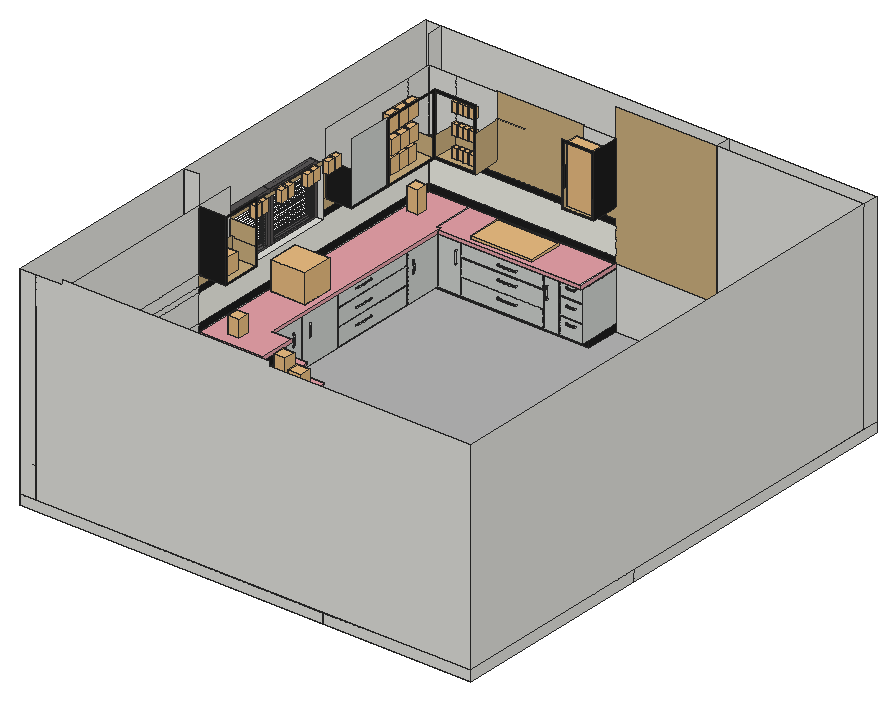
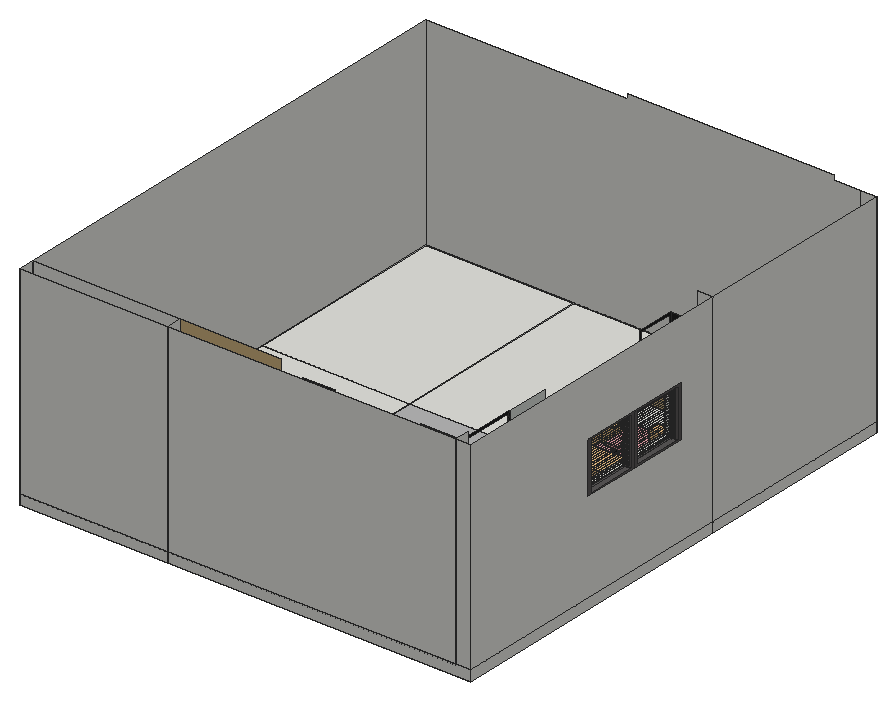
# SketchUp Ruby script. Lengths in inches.
U = 1.inch
M = Sketchup.active_model
def pt(a) = Geom::Point3d.new(a.map { |v| v * U })
def face(e, loops, mat)
  f = e.add_face(loops[0].map { |a| pt(a) })
  loops[1..].each { |l| e.add_face(l.map { |a| pt(a) }).erase! }
  f.material = f.back_material = mat if mat
  f
end
# faces: each face lists its corners as indices into pts; further lists are holes
def faces(e, pts, list, mat = nil) = list.each { |f| face(e, (f[0].is_a?(Array) ? f : [f]).map { |l| l.map { |i| pts[i] } }, mat) }
# xy, xz, yz: faces in a plane at the given z, y or x. An outline is a flat list of corners, or four numbers for a rectangle; further outlines are holes
def ring(l) = l.size == 4 ? [[l[0], l[1]], [l[2], l[1]], [l[2], l[3]], [l[0], l[3]]] : l.each_slice(2).to_a
def flat(e, list, mat, &to3) = list.each { |f| face(e, (f[0].is_a?(Array) ? f : [f]).map { |l| ring(l).map { |u, v| to3.(u, v) } }, mat) }
def xy(e, z, list, mat = nil) = flat(e, list, mat) { |x, y| [x, y, z] }
def xz(e, y, list, mat = nil) = flat(e, list, mat) { |x, z| [x, y, z] }
def yz(e, x, list, mat = nil) = flat(e, list, mat) { |y, z| [x, y, z] }
def lines(e, pts, list) = list.each { |a, b| e.add_line(pt(pts[a]), pt(pts[b])) }
# prism: a flat outline (further loops are holes) pulled along v
def prism(e, loops, v, mat = nil)
  f = face(e, loops, mat); d = Geom::Vector3d.new(v.map { |x| x * U })
  f.pushpull(f.normal.samedirection?(d) ? d.length : -d.length)
end
def box(e, o, s, mat = nil) = prism(e, [[o, [o[0] + s[0], o[1], o[2]], [o[0] + s[0], o[1] + s[1], o[2]], [o[0], o[1] + s[1], o[2]]]], [0, 0, s[2]], mat)
def at(x, y, z, deg = 0) = Geom::Transformation.translation(pt([x, y, z])) * Geom::Transformation.rotation(ORIGIN, Z_AXIS, deg.degrees)
def axes(o, x, y, z) = Geom::Transformation.new([*x, 0, *y, 0, *z, 0, *pt(o).to_a, 1])
def part(name) = M.definitions.add(name)
# library, detail: a bought-in or finely detailed component or shape, given as its bounding box
def library(name, o, s) = part(name).tap { |d| box(d.entities, o, s) }
def detail(e, o, s) = box(e.add_group.entities, o, s)
def put(e, d, t, mat = nil) = e.add_instance(d, t).tap { |i| i.material = mat if mat }
def group(e, t, mat = nil) = e.add_group.tap { |g| g.transformation = t; g.material = mat if mat }.entities
root = M.entities
M.materials.add("Emissive").color = [223, 214, 154]
M.materials.add("GLASS BLADE REFRACTION").color = [24, 24, 24]
M.materials["GLASS BLADE REFRACTION"].alpha = 0.5
M.materials.add("Generic").color = [208, 212, 208]
M.materials.add("JalousieFrame").color = [89, 86, 86]
M.materials.add("Tiles Simple 02 100cm").color = [183, 183, 183]
M.materials.add("W148Z538F75_NILAYA PACIFICA FD26008 ROLL F75").color = [242, 242, 233]
M.materials.add("W148Z583F75_NILAYA PACIFICA FD26054 ROLL F75").color = [231, 161, 169]
M.materials.add("[Color M08]").color = [30, 30, 30]
M.materials.add("[Color M08]1").color = [30, 30, 30]
M.materials.add("[Translucent_Glass_Blue]1").color = [0, 0, 0]
M.materials["[Translucent_Glass_Blue]1"].alpha = 0
M.materials.add("[Wood Floor Light]").color = [204, 176, 127]
c1 = part("Gruppo\#20")
prism(c1.entities,[[[0.51,10.14,0],[0.39,11.02,0],[0.07,11.02,0],[0.07,11.42,0],[0.79,11.42,0],[0.91,10.47,0],[1.01,9.52,0],[1.08,8.57,0],[1.14,7.62,0],[1.17,6.66,0],[1.18,5.71,0],[1.17,4.75,0],[1.14,3.8,0],[1.08,2.85,0],[1.01,1.9,0],[0.91,0.95,0],[0.79,0,0],[0,0,0],[0,0.39,0],[0.39,0.39,0],[0.51,1.27,0],[0.61,2.16,0],[0.6875,3.04,0],[0.74,3.93,0],[0.78,4.82,0],[0.79,5.71,0],[0.78,6.6,0],[0.74,7.49,0],[0.6875,8.375,0],[0.61,9.26,0]]],[0,0,0.39])
c2 = library("Potted Plant 50-23",[-3.4,-3.5,0],[6.8,7,9.93])
c3 = library("Group\#15",[179.9,72.7,378.72],[113.8,95.46,197.69])
c4 = library("Group\#16",[327.72,72.7,378.72],[113.79,95.46,197.69])
c5 = library("Group\#18",[-198.8,84.74,613.85],[84,84,172.39])
c6 = library("Group\#19",[-105.26,84.74,613.85],[84,84,172.39])
c7 = library("Group\#22",[-15.73,84.74,613.85],[84,84,172.39])
c8 = library("Group\#26",[85.42,84.74,613.85],[84,84,172.42])
c9 = library("Group\#30",[-504.125,120.57,-0.1],[108.2,108.21,338.13])
c10 = library("Group\#31",[-376.9,120.94,-0.1],[107.79,107.8,326.37])
c11 = library("Group\#32",[-254.81,120.48,-0.6],[108.21,108.21,334.5])
c12 = part("kitchen utensils3")
p = [[0,0,0],[1,0,0],[1,1,0]]
lines(c12.entities,p,[[0,1],[1,2],[2,0]])
put(c12.entities,c3,axes([15.76,143.39,56.31],[0,0.03485,0],[-0.03485,0,0],[0,0,0.03485]))
put(c12.entities,c4,axes([15.76,143.39,56.31],[0,0.03485,0],[-0.03485,0,0],[0,0,0.03485]))
put(c12.entities,c5,axes([32.2,277.71,52.16],[0.03485,0,0],[0,0.03485,0],[0,0,0.03485]))
put(c12.entities,c6,axes([32.2,277.71,52.16],[0.03485,0,0],[0,0.03485,0],[0,0,0.03485]))
put(c12.entities,c7,axes([32.2,277.71,52.16],[0.03485,0,0],[0,0.03485,0],[0,0,0.03485]))
put(c12.entities,c8,axes([32.2,277.71,52.16],[0.03485,0,0],[0,0.03485,0],[0,0,0.03485]))
put(c12.entities,c9,axes([18.2,277.99,72.21],[0,0.05935,0],[-0.03485,0,0],[0,0,0.02892]))
put(c12.entities,c10,axes([18.2,277.99,72.21],[0,0.05935,0],[-0.03485,0,0],[0,0,0.02892]))
put(c12.entities,c11,axes([18.2,277.99,72.21],[0,0.05935,0],[-0.03485,0,0],[0,0,0.02892]))
put(c12.entities,c5,axes([32.2,277.71,40.01],[0.03485,0,0],[0,0.03485,0],[0,0,0.03485]))
put(c12.entities,c6,axes([32.2,277.71,40.01],[0.03485,0,0],[0,0.03485,0],[0,0,0.03485]))
put(c12.entities,c7,axes([32.2,277.71,40.01],[0.03485,0,0],[0,0.03485,0],[0,0,0.03485]))
put(c12.entities,c8,axes([32.2,277.71,40.01],[0.03485,0,0],[0,0.03485,0],[0,0,0.03485]))
put(c12.entities,c5,axes([32.2,277.71,27.45],[0.03485,0,0],[0,0.03485,0],[0,0,0.03485]))
put(c12.entities,c8,axes([32.2,277.71,27.45],[0.03485,0,0],[0,0.03485,0],[0,0,0.03485]))
put(c12.entities,c7,axes([32.2,277.71,27.45],[0.03485,0,0],[0,0.03485,0],[0,0,0.03485]))
put(c12.entities,c6,axes([32.2,277.71,27.45],[0.03485,0,0],[0,0.03485,0],[0,0,0.03485]))
put(c12.entities,c11,axes([18.56,277.08,60.19],[0,0.05557,0],[-0.03485,0,0],[0,0,0.02506]))
put(c12.entities,c10,axes([18.56,277.08,60.19],[0,0.05557,0],[-0.03485,0,0],[0,0,0.02506]))
put(c12.entities,c9,axes([18.56,277.08,60.19],[0,0.05557,0],[-0.03485,0,0],[0,0,0.02506]))
put(c12.entities,c9,axes([17.31,276.63,48.84],[0,0.05174,0],[-0.03485,0,0],[0,0,0.02579]))
put(c12.entities,c10,axes([17.31,276.63,48.84],[0,0.05174,0],[-0.03485,0,0],[0,0,0.02579]))
put(c12.entities,c11,axes([17.31,276.63,48.84],[0,0.05174,0],[-0.03485,0,0],[0,0,0.02579]))
put(c12.entities,c4,axes([15.76,162.58,56.31],[0,0.03485,0],[-0.03485,0,0],[0,0,0.03485]))
put(c12.entities,c3,axes([15.76,162.58,56.31],[0,0.03485,0],[-0.03485,0,0],[0,0,0.03485]))
put(c12.entities,c4,axes([15.76,181.77,56.31],[0,0.03485,0],[-0.03485,0,0],[0,0,0.03485]))
put(c12.entities,c3,axes([15.76,181.77,56.31],[0,0.03485,0],[-0.03485,0,0],[0,0,0.03485]))
put(c12.entities,c3,axes([15.76,197.77,56.31],[0,0.03485,0],[-0.03485,0,0],[0,0,0.03485]))
put(c12.entities,c4,axes([15.76,197.77,56.31],[0,0.03485,0],[-0.03485,0,0],[0,0,0.03485]))
c13 = library("Interior Props 221 031",[-3.74,-3.52,-0.04],[7.48,7.03,11.78])
c14 = library("sink",[-18.39,0,-10.63],[18.4,20.47,27.45])
c15 = library("Utensils",[0,-0.54,-0.24],[6.34,6.28,13.37])
c16 = library("Bosch Stove",[0,0,0],[36.22,20.12,1.38])
c17 = part("Louvre end clip")
prism(c17.entities,[[[0,0.74,4.2],[0,0.38,4.24],[0,-0.06,-0.03],[0,0.29,-0.06],[0,0.3125,0.17],[0,0.26,0.18],[0,0.24,-0.02],[0,-0.02,0.01],[0,0.42,4.2],[0,0.68,4.17],[0,0.66,3.97],[0,0.71,3.97]]],[-0.59,0,0],"JalousieFrame")
c18 = part("Louvre blade")
xy(c18.entities,0,[[3.2,0,48.34,0.24]],"GLASS BLADE REFRACTION")
xy(c18.entities,4.17,[[3.2,0,48.34,0.24]],"GLASS BLADE REFRACTION")
xz(c18.entities,0,[[3.2,0,48.34,4.17]],"[Translucent_Glass_Blue]1")
xz(c18.entities,0.24,[[3.2,0,48.34,4.17]],"[Translucent_Glass_Blue]1")
yz(c18.entities,3.2,[[0,0,0.24,4.17]],"[Translucent_Glass_Blue]1")
yz(c18.entities,48.34,[[0,0,0.24,4.17]],"[Translucent_Glass_Blue]1")
c19 = part("Louvre blade assembly")
put(c19.entities,c17,axes([29.56,0.12,0.28],[1,0,0],[0,1.01433,-0.13582],[0,-0.20296,0.86161]))
put(c19.entities,c17,axes([1.96,0.12,0.28],[-1,0,0],[0,1.01433,-0.13582],[0,-0.20296,0.86161]))
put(c19.entities,c18,axes([0,0.12,0.3],[0.61176,0,0],[0,1.02999,-0.22514],[0,-0.09582,0.84269]))
c20 = part("Louvre blade assembly \#1")
put(c20.entities,c19,axes([-2.4,1.66,-0.39],[1.63462,0,0],[0,0.98741,-0.15853],[0,0.15779,0.98741]))
c21 = part("Group6\#2")
box(c21.entities,[-2.07,2.02,1.67],[0.98,0.98,67.72],"JalousieFrame")
c22 = part("Closed louvred window")
put(c22.entities,c20,axes([1.57,0.98,65.83],[0.61176,0,0],[0,1,0],[0,0,0.99766]))
put(c22.entities,c20,axes([1.57,0.98,62.79],[0.61176,0,0],[0,1,0],[0,0,0.99766]))
put(c22.entities,c20,axes([1.57,0.98,59.75],[0.61176,0,0],[0,1,0],[0,0,0.99766]))
put(c22.entities,c20,axes([1.57,0.98,56.7],[0.61176,0,0],[0,1,0],[0,0,0.99766]))
put(c22.entities,c20,axes([1.57,0.98,53.66],[0.61176,0,0],[0,1,0],[0,0,0.99766]))
put(c22.entities,c20,axes([1.57,0.98,50.61],[0.61176,0,0],[0,1,0],[0,0,0.99766]))
put(c22.entities,c20,axes([1.57,0.98,47.57],[0.61176,0,0],[0,1,0],[0,0,0.99766]))
put(c22.entities,c20,axes([1.57,0.98,44.53],[0.61176,0,0],[0,1,0],[0,0,0.99766]))
put(c22.entities,c20,axes([1.57,0.98,41.48],[0.61176,0,0],[0,1,0],[0,0,0.99766]))
put(c22.entities,c20,axes([1.57,0.98,38.4375],[0.61176,0,0],[0,1,0],[0,0,0.99766]))
put(c22.entities,c20,axes([1.57,0.98,35.39],[0.61176,0,0],[0,1,0],[0,0,0.99766]))
put(c22.entities,c20,axes([1.57,0.98,32.35],[0.61176,0,0],[0,1,0],[0,0,0.99766]))
put(c22.entities,c20,axes([1.57,0.98,29.31],[0.61176,0,0],[0,1,0],[0,0,0.99766]))
put(c22.entities,c20,axes([1.57,0.98,26.26],[0.61176,0,0],[0,1,0],[0,0,0.99766]))
put(c22.entities,c20,axes([1.57,0.98,23.22],[0.61176,0,0],[0,1,0],[0,0,0.99766]))
put(c22.entities,c20,axes([1.57,0.98,20.17],[0.61176,0,0],[0,1,0],[0,0,0.99766]))
put(c22.entities,c20,axes([1.57,0.98,17.13],[0.61176,0,0],[0,1,0],[0,0,0.99766]))
put(c22.entities,c20,axes([1.57,0.98,14.09],[0.61176,0,0],[0,1,0],[0,0,0.99766]))
put(c22.entities,c20,axes([1.57,0.98,11.04],[0.61176,0,0],[0,1,0],[0,0,0.99766]))
put(c22.entities,c20,axes([1.57,0.98,8],[0.61176,0,0],[0,1,0],[0,0,0.99766]))
put(c22.entities,c20,axes([1.57,0.98,4.95],[0.61176,0,0],[0,1,0],[0,0,0.99766]))
put(c22.entities,c20,axes([1.57,0.98,1.91],[0.61176,0,0],[0,1,0],[0,0,0.99766]))
g1 = group(c22.entities,at(0,0.98,0.1))
xy(g1,0,[[0,0.1,31.72,4.92]],"JalousieFrame")
xy(g1,1.57,[[1.57,0.1,30.15,4.92]],"JalousieFrame")
xy(g1,69.29,[[1.57,0.1,30.15,4.92]],"JalousieFrame")
xy(g1,70.87,[[0,0.1,31.72,4.92]],"JalousieFrame")
xz(g1,0,[[[0.1,0.1,31.625,70.77],[1.47,1.48,30.25,69.39]]],"JalousieFrame")
xz(g1,4.92,[[[0,0,31.72,70.87],[1.57,1.57,30.15,69.29]]],"JalousieFrame")
yz(g1,0,[[0.1,0,4.92,70.87]],"JalousieFrame")
yz(g1,1.57,[[0.1,1.57,4.92,69.29]],"JalousieFrame")
yz(g1,30.15,[[0.1,1.57,4.92,69.29]],"JalousieFrame")
yz(g1,31.72,[[0.1,0,4.92,70.87]],"JalousieFrame")
p = [[0,0.1,70.87],[0,0.1,0],[0.1,0,0.1],[0.1,0,70.77],[31.72,0.1,0],[31.625,0,0.1],
  [31.72,0.1,70.87],[31.625,0,70.77],[30.15,0.1,1.57],[1.57,0.1,1.57],[1.47,0,1.48],[30.25,0,1.48],
  [1.57,0.1,69.29],[1.47,0,69.39],[30.15,0.1,69.29],[30.25,0,69.39]]
faces(g1,p,[[0,1,2,3],[1,4,5,2],[4,6,7,5],[8,9,10,11],[9,12,13,10],[14,8,11,15],[12,14,15,13],[6,0,3,7]],"JalousieFrame")
put(c22.entities,c21,axes([31.72,0.98,0],[0.99482,0,0],[0,1,0],[0,0,1]))
put(c22.entities,c21,axes([0,0.98,0],[-0.99482,0,0],[0,1,0],[0,0,1]))
c23 = part("Louvre blade assembly \#2")
put(c23.entities,c19,axes([-2.4,0.24,0.625],[1.63462,0,0],[0,0.5,-0.86805],[0,0.864,0.5]))
c24 = part("Group6\#1")
box(c24.entities,[-2.07,2.02,1.67],[0.98,0.98,67.72],"JalousieFrame")
c25 = part("Open louvred window")
put(c25.entities,c23,axes([1.57,0.98,65.83],[0.61176,0,0],[0,1,0],[0,0,0.99766]))
put(c25.entities,c23,axes([1.57,0.98,62.79],[0.61176,0,0],[0,1,0],[0,0,0.99766]))
put(c25.entities,c23,axes([1.57,0.98,59.75],[0.61176,0,0],[0,1,0],[0,0,0.99766]))
put(c25.entities,c23,axes([1.57,0.98,56.7],[0.61176,0,0],[0,1,0],[0,0,0.99766]))
put(c25.entities,c23,axes([1.57,0.98,53.66],[0.61176,0,0],[0,1,0],[0,0,0.99766]))
put(c25.entities,c23,axes([1.57,0.98,50.61],[0.61176,0,0],[0,1,0],[0,0,0.99766]))
put(c25.entities,c23,axes([1.57,0.98,47.57],[0.61176,0,0],[0,1,0],[0,0,0.99766]))
put(c25.entities,c23,axes([1.57,0.98,44.53],[0.61176,0,0],[0,1,0],[0,0,0.99766]))
put(c25.entities,c23,axes([1.57,0.98,41.48],[0.61176,0,0],[0,1,0],[0,0,0.99766]))
put(c25.entities,c23,axes([1.57,0.98,38.4375],[0.61176,0,0],[0,1,0],[0,0,0.99766]))
put(c25.entities,c23,axes([1.57,0.98,35.39],[0.61176,0,0],[0,1,0],[0,0,0.99766]))
put(c25.entities,c23,axes([1.57,0.98,32.35],[0.61176,0,0],[0,1,0],[0,0,0.99766]))
put(c25.entities,c23,axes([1.57,0.98,29.31],[0.61176,0,0],[0,1,0],[0,0,0.99766]))
put(c25.entities,c23,axes([1.57,0.98,26.26],[0.61176,0,0],[0,1,0],[0,0,0.99766]))
put(c25.entities,c23,axes([1.57,0.98,23.22],[0.61176,0,0],[0,1,0],[0,0,0.99766]))
put(c25.entities,c23,axes([1.57,0.98,20.17],[0.61176,0,0],[0,1,0],[0,0,0.99766]))
put(c25.entities,c23,axes([1.57,0.98,17.13],[0.61176,0,0],[0,1,0],[0,0,0.99766]))
put(c25.entities,c23,axes([1.57,0.98,14.09],[0.61176,0,0],[0,1,0],[0,0,0.99766]))
put(c25.entities,c23,axes([1.57,0.98,11.04],[0.61176,0,0],[0,1,0],[0,0,0.99766]))
put(c25.entities,c23,axes([1.57,0.98,8],[0.61176,0,0],[0,1,0],[0,0,0.99766]))
put(c25.entities,c23,axes([1.57,0.98,4.95],[0.61176,0,0],[0,1,0],[0,0,0.99766]))
put(c25.entities,c23,axes([1.57,0.98,1.91],[0.61176,0,0],[0,1,0],[0,0,0.99766]))
g2 = group(c25.entities,at(0,0.98,0.1))
xy(g2,0,[[0,0.1,31.72,4.92]],"JalousieFrame")
xy(g2,1.57,[[1.57,0.1,30.15,4.92]],"JalousieFrame")
xy(g2,69.29,[[1.57,0.1,30.15,4.92]],"JalousieFrame")
xy(g2,70.87,[[0,0.1,31.72,4.92]],"JalousieFrame")
xz(g2,0,[[[0.1,0.1,31.625,70.77],[1.47,1.48,30.25,69.39]]],"JalousieFrame")
xz(g2,4.92,[[[0,0,31.72,70.87],[1.57,1.57,30.15,69.29]]],"JalousieFrame")
yz(g2,0,[[0.1,0,4.92,70.87]],"JalousieFrame")
yz(g2,1.57,[[0.1,1.57,4.92,69.29]],"JalousieFrame")
yz(g2,30.15,[[0.1,1.57,4.92,69.29]],"JalousieFrame")
yz(g2,31.72,[[0.1,0,4.92,70.87]],"JalousieFrame")
p = [[0,0.1,70.87],[0,0.1,0],[0.1,0,0.1],[0.1,0,70.77],[31.72,0.1,0],[31.625,0,0.1],
  [31.72,0.1,70.87],[31.625,0,70.77],[30.15,0.1,1.57],[1.57,0.1,1.57],[1.47,0,1.48],[30.25,0,1.48],
  [1.57,0.1,69.29],[1.47,0,69.39],[30.15,0.1,69.29],[30.25,0,69.39]]
faces(g2,p,[[0,1,2,3],[1,4,5,2],[4,6,7,5],[8,9,10,11],[9,12,13,10],[14,8,11,15],[12,14,15,13],[6,0,3,7]],"JalousieFrame")
put(c25.entities,c24,axes([31.72,0.98,0],[0.99482,0,0],[0,1,0],[0,0,1]))
put(c25.entities,c24,axes([0,0.98,0],[-0.99482,0,0],[0,1,0],[0,0,1]))
c26 = part("JSilva Jalousie")
put(c26.entities,c22,axes([0,-0.98,0],[-1.0052,0,0],[0,1,0],[0,0,1]))
put(c26.entities,c25,axes([31.89,-0.98,0],[-1.0052,0,0],[0,1,0],[0,0,1]))
c27 = library("Glass_Apothecary_Jar",[-12.71,110.07,67],[15.12,7.6,33.89])
xy(root,-6,[[0.32,0,180.32,121.64],[180.32,0,268.26,121.64],[0.32,121.64,180.32,301.64],[180.32,121.64,268.26,301.64]])
xy(root,0,[[0.32,0,9.32,121.64],[9.32,0,68.51,121.64],[68.51,0,180.32,121.64],[180.32,0,268.26,121.64],[0.32,121.64,9.32,301.64],
  [9.32,121.64,68.51,121.64,68.51,137.13,29.32,137.13,29.32,272.64,33.32,272.64,33.32,292.64,9.32,292.64],[180.32,121.64,268.26,292.64],[33.32,272.64,120.26,292.64],[33.32,272.64,120.26,292.64],[9.32,292.64,180.32,301.64],
  [180.32,292.64,268.26,301.64]])
xy(root,0,[[68.51,121.64,180.32,121.64,180.32,292.64,120.26,292.64,120.26,272.64,29.32,272.64,29.32,137.13,68.51,137.13]],"Tiles Simple 02 100cm")
xy(root,4,[[9.32,121.64,9.32,292.64,33.32,292.64,33.32,272.64,29.32,272.64,29.32,137.13,68.51,137.13,68.51,121.64],[69.57,121.64,69.57,138,30.01,138,30.01,272.18,106.34,272.18,106.34,268.64,33.32,268.64,33.32,141.13,74.29,141.13,74.47,141.125,74.64,141.1,74.81,141.06,74.97,141,75.13,140.93,75.28,140.84,75.42,140.74,75.55,140.625,75.67,140.5,75.78,140.36,75.87,140.22,75.95,140.0625,75.95,122.9375,75.85,122.75,75.74,122.57,75.61,122.41,75.47,122.25,75.31,122.11,75.14,121.99,74.96,121.88,74.76,121.8,74.57,121.73,74.36,121.68,74.15,121.65,73.94,121.64],[33.32,272.64,120.26,292.64]])
xy(root,4,[[106.34,268.64,119.86,272.18],[119.86,268.64,120.26,272.18],[106.34,272.18,119.86,272.64],[119.86,272.18,120.26,272.64]],"[Color M08]")
xy(root,4.1875,[[68.51,121.64,68.51,137.13,29.32,137.13,29.32,272.64,106.34,272.64,106.34,272.18,30.01,272.18,30.01,138,69.57,138,69.57,121.64]],"Emissive")
xy(root,11.25,[[66.51,121.64,66.51,141.13,74.29,141.13,74.47,141.125,74.64,141.1,74.81,141.06,74.97,141,75.13,140.93,75.28,140.84,75.42,140.74,75.55,140.625,75.67,140.5,75.78,140.36,75.87,140.22,75.95,140.0625,75.95,122.9375,75.85,122.75,75.74,122.57,75.61,122.41,75.47,122.25,75.31,122.11,75.14,121.99,74.96,121.88,74.76,121.8,74.57,121.73,74.36,121.68,74.15,121.65,73.94,121.64]])
xy(root,11.25,[[66.51,119.64,75.95,121.64],[75.95,119.64,75.95,143.13,76.55,141.23,77.05,139.3,77.44,137.34,77.72,135.37,77.89,133.38,77.95,131.38,77.89,129.39,77.72,127.4,77.44,125.43,77.05,123.47,76.55,121.54],[66.51,141.13,75.95,143.13]],"W148Z583F75_NILAYA PACIFICA FD26054 ROLL F75")
xy(root,12.25,[[66.51,119.64,75.95,119.64,76.55,121.54,77.05,123.47,77.44,125.43,77.72,127.4,77.89,129.39,77.95,131.38,77.89,133.38,77.72,135.37,77.44,137.34,77.05,139.3,76.55,141.23,75.95,143.13,66.51,143.13]],"W148Z583F75_NILAYA PACIFICA FD26054 ROLL F75")
xy(root,18.5,[[56.45,121.64,66.51,141.13]])
xy(root,18.5,[[56.45,119.64,66.51,121.64],[66.51,119.64,66.51,143.13,67.12,141.23,67.62,139.3,68.01,137.34,68.29,135.37,68.45,133.38,68.51,131.38,68.45,129.39,68.29,127.4,68.01,125.43,67.62,123.47,67.12,121.54],[56.45,141.13,66.51,143.13]],"W148Z583F75_NILAYA PACIFICA FD26054 ROLL F75")
xy(root,19.5,[[56.45,119.64,66.51,119.64,67.12,121.54,67.62,123.47,68.01,125.43,68.29,127.4,68.45,129.39,68.51,131.38,68.45,133.38,68.29,135.37,68.01,137.34,67.62,139.3,67.12,141.23,66.51,143.13,56.45,143.13]],"W148Z583F75_NILAYA PACIFICA FD26054 ROLL F75")
xy(root,25.75,[[45.14,121.64,56.45,141.13]])
xy(root,25.75,[[56.45,121.64,56.45,143.13,57.05,141.4,57.55,139.64,57.94,137.85,58.22,136.04,58.39,134.22,58.45,132.38,58.39,130.55,58.22,128.73,57.94,126.92,57.55,125.13,57.05,123.37],[45.14,141.13,56.45,143.13]],"W148Z583F75_NILAYA PACIFICA FD26054 ROLL F75")
xy(root,27,[[45.14,121.64,56.45,121.64,57.05,123.37,57.55,125.13,57.94,126.92,58.22,128.73,58.39,130.55,58.45,132.38,58.39,134.22,58.22,136.04,57.94,137.85,57.55,139.64,57.05,141.4,56.45,143.13,45.14,143.13]],"W148Z583F75_NILAYA PACIFICA FD26054 ROLL F75")
xy(root,33,[[33.32,268.64,120.26,292.64]])
xy(root,34,[[[9.32,121.64,9.32,292.64,33.32,292.64,33.32,141.13,45.14,141.13,45.14,121.64],[11.25,172.64,31.55,191.03]],[33.32,268.64,120.26,292.64]])
xy(root,34,[[45.14,121.64,47.14,143.13],[33.32,141.13,45.14,143.13],[33.32,143.13,35.32,268.64],[35.32,266.64,120.26,268.64]],"W148Z583F75_NILAYA PACIFICA FD26054 ROLL F75")
xy(root,36,[[119.86,266.64,120.26,292.64]])
xy(root,36,[[[9.32,121.64,47.14,121.64,47.14,143.13,35.32,143.13,35.32,268.64,33.32,268.64,33.32,292.64,9.32,292.64],[11.25,172.64,31.55,191.03]],[35.32,266.64,119.86,266.64,119.86,292.64,33.32,292.64,33.32,268.64,35.32,268.64]],"W148Z583F75_NILAYA PACIFICA FD26054 ROLL F75")
xy(root,54.78,[[0.32,145.89,9.32,214.64]])
xy(root,66,[[10.32,121.64,25.32,144.53],[10.32,215.6,10.32,291.64,49.83,291.64,49.83,276.64,25.32,276.64,25.32,215.6],[101.36,276.64,120.26,291.64]],"[Color M08]")
xy(root,66.75,[[9.32,121.64,10.32,144.53],[9.32,215.6,9.32,292.64,49.83,292.64,49.83,291.64,10.32,291.64,10.32,215.6],[101.36,291.64,120.26,292.64]],"Emissive")
xy(root,67,[[11.32,122.64,25.32,143.53],[11.32,242.875,25.32,275.64],[26.32,276.64,48.83,290.64],[102.36,276.64,119.26,290.64]],"[Wood Floor Light]")
xz(root,0,[[0.32,-6,180.32,0],[180.32,-6,268.26,0],[0.32,0,9.32,120],[9.32,0,268.26,0,268.26,120,148.26,120,148.26,123,25.32,123,25.32,120,9.32,120]])
xz(root,119.64,[[66.51,11.25,75.95,12.25],[56.45,18.5,66.51,19.5]],"W148Z583F75_NILAYA PACIFICA FD26054 ROLL F75")
xz(root,121.64,[[0.32,-6,180.32,0],[180.32,-6,268.26,0],[0.32,0,9.32,120],[9.32,33,45.14,34]])
xz(root,121.64,[[9.32,4,68.51,4,68.51,4.1875,69.57,4.1875,69.57,4,73.94,4,73.94,11.25,66.51,11.25,66.51,18.5,56.45,18.5,56.45,25.75,45.14,25.75,45.14,33,9.32,33]],"W148Z538F75_NILAYA PACIFICA FD26008 ROLL F75")
xz(root,121.64,[[45.14,25.75,56.45,27],[9.32,34,47.14,36]],"W148Z583F75_NILAYA PACIFICA FD26054 ROLL F75")
xz(root,121.64,[[9.32,0,68.51,4],[10.32,66,25.32,66,25.32,103.04,9.32,103.04,9.32,66.75,10.32,66.75]],"[Color M08]")
xz(root,122.64,[[11.32,67,11.32,78.07,12.32,78.07,12.32,77.32,25.32,77.32,25.32,67]],"[Wood Floor Light]")
xz(root,137.13,[[29.32,0,68.51,4]])
xz(root,137.13,[[29.32,4,68.51,4.1875]],"Emissive")
xz(root,138,[[30.01,4,69.57,4.1875]],"Emissive")
xz(root,141.13,[[33.32,4,74.29,11.25],[33.32,11.25,66.51,18.5],[33.32,18.5,56.45,25.75],[33.32,25.75,45.14,33],[33.32,33,45.14,34]],"[Color M08]")
xz(root,143.13,[[66.51,11.25,75.95,12.25],[56.45,18.5,66.51,19.5],[45.14,25.75,56.45,27],[35.32,34,47.14,36]],"W148Z583F75_NILAYA PACIFICA FD26054 ROLL F75")
xz(root,143.53,[[11.32,67,25.32,67,25.32,77.32,12.32,77.32,12.32,78.07,11.32,78.07]],"[Wood Floor Light]")
xz(root,144.53,[[10.32,66,10.32,66.75,9.32,66.75,9.32,86.75,25.32,86.75,25.32,66]],"[Wood Floor Light]")
xz(root,145.89,[[0.32,54.78,9.32,66],[0.32,66,9.32,84.97]])
xz(root,172.64,[[11.25,34,31.55,36]],"W148Z583F75_NILAYA PACIFICA FD26054 ROLL F75")
xz(root,191.03,[[11.25,34,31.55,36]],"W148Z583F75_NILAYA PACIFICA FD26054 ROLL F75")
xz(root,214.64,[[0.32,54.78,9.32,84.97]])
xz(root,215.6,[[10.32,66,25.32,66,25.32,86.75,9.32,86.75,9.32,66.75,10.32,66.75]],"[Color M08]")
xz(root,242.875,[[11.32,67,11.32,78.3125,12.32,78.3125,12.32,77.5625,25.32,77.5625,25.32,67]],"[Wood Floor Light]")
xz(root,266.64,[[35.32,34,120.26,36]],"W148Z583F75_NILAYA PACIFICA FD26054 ROLL F75")
xz(root,268.64,[[119.86,14.15,119.89,24.7],[33.32,34,35.32,36]])
xz(root,268.64,[[33.72,4,47.35,33],[47.75,4,96.49,14.15],[96.89,4,105.94,33],[106.34,4,119.86,4,119.86,14.15,106.37,14.15,106.37,14.55,106.34,14.55],[47.75,14.55,96.49,24.7],
  [106.37,14.55,119.86,24.7],[47.75,25.1,96.49,33],[106.34,25.1,119.86,33]],"Generic")
xz(root,268.64,[[33.32,4,33.72,33],[47.35,4,47.75,33],[96.49,4,96.89,33],[105.94,4,106.34,33],[119.86,4,120.26,4,120.26,33,119.86,33,119.86,24.7,119.89,24.7,119.89,14.15,119.86,14.15],
  [47.75,14.15,96.49,14.55],[106.37,14.15,119.86,14.55],[106.34,14.55,106.37,14.55,106.37,24.7,119.86,24.7,119.86,25.1,106.34,25.1],[47.75,24.7,96.49,25.1],[33.32,33,120.26,34]],"[Color M08]")
xz(root,272.18,[[30.01,4,106.34,4.1875]],"Emissive")
xz(root,272.64,[[29.32,4,33.32,4.1875],[33.32,4,106.34,4.1875]],"Emissive")
xz(root,272.64,[[29.32,0,33.32,4],[33.32,0,120.26,4]],"[Color M08]")
xz(root,275.64,[[11.32,67,25.32,67,25.32,77.5625,12.32,77.5625,12.32,78.3125,11.32,78.3125]],"[Wood Floor Light]")
xz(root,276.64,[[[25.32,66,49.83,103.04],[26.32,67,48.83,102.04]],[[101.36,66,120.26,103.04],[102.36,67,119.26,102.04]]],"[Color M08]")
xz(root,290.64,[[26.32,67,48.83,79.45],[102.36,67,119.26,77.87]],"[Wood Floor Light]")
xz(root,291.64,[[10.32,66,49.83,66.75],[101.36,66,120.26,66.75]],"Emissive")
xz(root,292.64,[[9.32,0,33.32,4],[33.32,0,120.26,4],[120.26,0,180.32,36],[180.32,0,268.26,36],[9.32,4,33.32,33],
  [33.32,4,120.26,33],[9.32,33,33.32,34],[33.32,33,120.26,34],[9.32,34,33.32,36],[33.32,34,120.26,36],
  [180.32,36,268.26,120],[9.32,66.75,25.32,103.04],[25.32,66.75,49.83,103.04],[101.36,66.75,120.26,103.04]])
xz(root,292.64,[[120.26,40.125,120.26,56.6875,9.32,56.6875,9.32,40.1875]],"W148Z538F75_NILAYA PACIFICA FD26008 ROLL F75")
xz(root,292.64,[[9.32,36,120.26,36,120.26,40.125,9.32,40.1875],[9.32,56.6875,120.26,60]],"[Color M08]")
xz(root,292.64,[[120.26,36,180.32,36,180.32,120,120.26,120,120.26,66.75,101.36,66.75,101.36,88.75,85.24,88.75,85.24,88.9375,101.36,88.9375,101.36,103.79,49.83,103.79,49.83,89.1,66.66,89.1,66.66,88.67,49.83,88.67,49.83,66.75,9.32,66.75,9.32,60,120.26,60]],"[Wood Floor Light]")
xz(root,301.64,[[0.32,-6,180.32,0],[180.32,-6,268.26,0],[0.32,0,9.32,120],[9.32,0,180.32,120],[180.32,0,268.26,120]])
yz(root,0.32,[[0,-6,121.64,0],[121.64,-6,301.64,0],[0,0,121.64,120],[[121.64,0,301.64,120],[145.89,54.78,214.64,84.97]]])
yz(root,9.32,[[0,0,121.64,4],[121.64,0,292.64,4],[292.64,0,301.64,120],[0,4,121.64,33],[121.64,4,292.64,33],
  [0,33,121.64,34],[121.64,33,292.64,34],[0,34,121.64,36],[121.64,34,292.64,36],[0,36,121.64,40.1875],
  [0,40.1875,121.64,56.6875],[0,56.6875,121.64,60],[0,60,121.64,66.75],[0,66.75,121.64,103.04],[121.64,66.75,144.53,103.04],
  [215.6,66.75,276.64,103.04],[276.64,66.75,292.64,103.04]])
yz(root,9.32,[[121.64,40.1875,292.64,40.1875,292.64,56.6875,214.64,56.6875,214.64,54.78,145.89,54.78,145.89,56.6875,121.64,56.6875]],"W148Z538F75_NILAYA PACIFICA FD26008 ROLL F75")
yz(root,9.32,[[121.64,36,292.64,40.1875],[121.64,56.6875,145.89,60],[214.64,56.6875,292.64,60]],"[Color M08]")
yz(root,9.32,[[121.64,60,145.89,60,145.89,66,144.53,66,144.53,66.75,121.64,66.75],[214.64,60,292.64,60,292.64,66.75,215.6,66.75,215.6,66,214.64,66],[144.53,66,145.89,66,145.89,84.97,214.64,84.97,214.64,66,215.6,66,215.6,86.75,144.53,86.75]],"[Wood Floor Light]")
yz(root,10.32,[[121.64,66,144.53,66.75],[215.6,66,291.64,66.75]],"Emissive")
yz(root,11.25,[[172.64,34,191.03,36]],"W148Z583F75_NILAYA PACIFICA FD26054 ROLL F75")
yz(root,11.32,[[122.64,67,143.53,78.07],[242.875,67,275.64,78.3125]],"[Wood Floor Light]")
yz(root,25.32,[[215.6,67.0625,241.48,103.04]],"Generic")
yz(root,25.32,[[[121.64,66,144.53,103.04],[122.64,67,143.53,102.04]],[215.6,66,241.875,67.0625],[[241.875,66,276.64,103.04],[242.875,67,275.64,102.04]],[241.48,67.0625,241.875,103.04]],"[Color M08]")
yz(root,26.32,[[276.64,67,290.64,67,290.64,79.45,289.64,79.45,289.64,78.7,276.64,78.7]],"[Wood Floor Light]")
yz(root,29.32,[[137.13,4,272.64,4.1875]],"Emissive")
yz(root,29.32,[[137.13,0,272.64,4]],"[Color M08]")
yz(root,30.01,[[138,4,272.18,4.1875]],"Emissive")
yz(root,31.55,[[172.64,34,191.03,36]],"W148Z583F75_NILAYA PACIFICA FD26054 ROLL F75")
yz(root,33.32,[[272.64,0,292.64,4],[268.64,33,292.64,34],[268.64,34,292.64,36]])
yz(root,33.32,[[141.13,4,167.72,33],[168.12,4,194.71,33],[195.11,4,246.4,14.15],[246.8,4,268.64,33],[195.11,14.55,246.4,24.7],
  [195.11,25.1,246.4,33]],"Generic")
yz(root,33.32,[[167.72,4,168.12,33],[194.71,4,195.11,33],[246.4,4,246.8,25.1],[195.11,14.15,246.4,14.55],[195.11,24.7,246.4,25.1],
  [246.4,25.1,246.8,33],[141.13,33,268.64,34]],"[Color M08]")
yz(root,35.32,[[266.64,34,268.64,36]])
yz(root,35.32,[[143.13,34,266.64,36]],"W148Z583F75_NILAYA PACIFICA FD26054 ROLL F75")
yz(root,45.14,[[121.64,25.75,141.13,27],[141.13,25.75,143.13,27]])
yz(root,45.14,[[121.64,27,141.13,34]],"[Color M08]")
yz(root,47.14,[[121.64,34,143.13,36]],"W148Z583F75_NILAYA PACIFICA FD26054 ROLL F75")
yz(root,48.83,[[276.64,67,276.64,78.7,289.64,78.7,289.64,79.45,290.64,79.45,290.64,67]],"[Wood Floor Light]")
yz(root,49.83,[[276.64,66,291.64,66,291.64,66.75,292.64,66.75,292.64,88.67,291.64,88.67,291.64,87.92,276.64,87.92]],"[Wood Floor Light]")
yz(root,56.45,[[119.64,18.5,121.64,19.5],[121.64,18.5,141.13,19.5],[141.13,18.5,143.13,19.5]])
yz(root,56.45,[[121.64,19.5,141.13,25.75]],"[Color M08]")
yz(root,66.51,[[119.64,11.25,121.64,12.25],[121.64,11.25,141.13,12.25],[141.13,11.25,143.13,12.25]])
yz(root,66.51,[[121.64,12.25,141.13,18.5]],"[Color M08]")
yz(root,68.51,[[121.64,4,137.13,4.1875]],"Emissive")
yz(root,68.51,[[121.64,0,137.13,4]],"[Color M08]1")
yz(root,69.57,[[121.64,4,138,4.1875]],"Emissive")
yz(root,75.95,[[122.9375,4,140.0625,11.25]],"[Color M08]")
yz(root,101.36,[[276.64,66,276.64,88,291.64,88,291.64,88.75,292.64,88.75,292.64,66.75,291.64,66.75,291.64,66]],"[Color M08]")
yz(root,102.36,[[276.64,67,290.64,67,290.64,77.87,289.64,77.87,289.64,77.12,276.64,77.12]],"[Wood Floor Light]")
yz(root,106.34,[[272.18,4,272.64,4.1875]],"Emissive")
yz(root,119.26,[[276.64,67,276.64,77.12,289.64,77.12,289.64,77.87,290.64,77.87,290.64,67]],"[Wood Floor Light]")
yz(root,120.26,[[268.64,4,292.64,33]],"Generic")
yz(root,120.26,[[266.64,34,292.64,36]],"W148Z583F75_NILAYA PACIFICA FD26054 ROLL F75")
yz(root,120.26,[[272.64,0,292.64,4],[268.64,33,292.64,34],[276.64,66,291.64,66,291.64,66.75,292.64,66.75,292.64,103.04,276.64,103.04]],"[Color M08]")
yz(root,180.32,[[0,-6,121.64,0],[121.64,-6,301.64,0],[292.64,0,301.64,120]])
yz(root,268.26,[[0,-6,121.64,0],[121.64,-6,301.64,0],[0,0,292.64,120],[292.64,0,301.64,120]])
p = [[73.94,121.64,4],[74.15,121.65,4],[74.15,121.65,11.25],[73.94,121.64,11.25],[74.36,121.68,4],[74.36,121.68,11.25],
  [74.57,121.73,4],[74.57,121.73,11.25],[74.76,121.8,4],[74.76,121.8,11.25],[74.96,121.88,4],[74.96,121.88,11.25],
  [75.14,121.99,4],[75.14,121.99,11.25],[75.31,122.11,4],[75.31,122.11,11.25],[75.47,122.25,4],[75.47,122.25,11.25],
  [75.61,122.41,4],[75.61,122.41,11.25],[75.74,122.57,4],[75.74,122.57,11.25],[75.85,122.75,4],[75.85,122.75,11.25],
  [75.95,122.9375,4],[75.95,122.9375,11.25],[75.95,140.0625,4],[75.87,140.22,4],[75.87,140.22,11.25],[75.95,140.0625,11.25],
  [75.78,140.36,4],[75.78,140.36,11.25],[75.67,140.5,4],[75.67,140.5,11.25],[75.55,140.625,4],[75.55,140.625,11.25],
  [75.42,140.74,4],[75.42,140.74,11.25],[75.28,140.84,4],[75.28,140.84,11.25],[75.13,140.93,4],[75.13,140.93,11.25],
  [74.97,141,4],[74.97,141,11.25],[74.81,141.06,4],[74.81,141.06,11.25],[74.47,141.125,4],[74.29,141.13,4],
  [74.29,141.13,11.25],[74.47,141.125,11.25],[74.64,141.1,4],[74.64,141.1,11.25],[76.55,121.54,12.25],[75.95,119.64,12.25],
  [75.95,119.64,11.25],[76.55,121.54,11.25],[77.05,123.47,12.25],[77.05,123.47,11.25],[77.44,125.43,12.25],[77.44,125.43,11.25],
  [77.72,127.4,12.25],[77.72,127.4,11.25],[77.89,129.39,12.25],[77.89,129.39,11.25],[77.95,131.38,12.25],[77.95,131.38,11.25],
  [77.89,133.38,12.25],[77.89,133.38,11.25],[77.72,135.37,12.25],[77.72,135.37,11.25],[77.44,137.34,12.25],[77.44,137.34,11.25],
  [77.05,139.3,12.25],[77.05,139.3,11.25],[76.55,141.23,12.25],[76.55,141.23,11.25],[75.95,143.13,12.25],[75.95,143.13,11.25],
  [67.12,121.54,19.5],[66.51,119.64,19.5],[66.51,119.64,18.5],[67.12,121.54,18.5],[67.62,123.47,19.5],[67.62,123.47,18.5],
  [68.01,125.43,19.5],[68.01,125.43,18.5],[68.29,127.4,19.5],[68.29,127.4,18.5],[68.45,129.39,19.5],[68.45,129.39,18.5],
  [68.51,131.38,19.5],[68.51,131.38,18.5],[68.45,133.38,19.5],[68.45,133.38,18.5],[68.29,135.37,19.5],[68.29,135.37,18.5],
  [68.01,137.34,19.5],[68.01,137.34,18.5],[67.62,139.3,19.5],[67.62,139.3,18.5],[67.12,141.23,19.5],[67.12,141.23,18.5],
  [66.51,143.13,19.5],[66.51,143.13,18.5],[57.05,123.37,27],[56.45,121.64,27],[56.45,121.64,25.75],[57.05,123.37,25.75],
  [57.55,125.13,27],[57.55,125.13,25.75],[57.94,126.92,27],[57.94,126.92,25.75],[58.22,128.73,27],[58.22,128.73,25.75],
  [58.39,130.55,27],[58.39,130.55,25.75],[58.45,132.38,27],[58.45,132.38,25.75],[58.39,134.22,27],[58.39,134.22,25.75],
  [58.22,136.04,27],[58.22,136.04,25.75],[57.94,137.85,27],[57.94,137.85,25.75],[57.55,139.64,27],[57.55,139.64,25.75],
  [57.05,141.4,27],[57.05,141.4,25.75],[56.45,143.13,27],[56.45,143.13,25.75]]
faces(root,p,[[0,1,2,3],[1,4,5,2],[4,6,7,5],[6,8,9,7],[8,10,11,9],[10,12,13,11],[12,14,15,13],[14,16,17,15],
  [16,18,19,17],[18,20,21,19],[20,22,23,21],[22,24,25,23],[26,27,28,29],[27,30,31,28],[30,32,33,31],[32,34,35,33],
  [34,36,37,35],[36,38,39,37],[38,40,41,39],[40,42,43,41],[42,44,45,43],[46,47,48,49],[50,46,49,51],[44,50,51,45]],"[Color M08]")
faces(root,p,[[52,53,54,55],[56,52,55,57],[58,56,57,59],[60,58,59,61],[62,60,61,63],[64,62,63,65],[66,64,65,67],[68,66,67,69],
  [70,68,69,71],[72,70,71,73],[74,72,73,75],[76,74,75,77],[78,79,80,81],[82,78,81,83],[84,82,83,85],[86,84,85,87],
  [88,86,87,89],[90,88,89,91],[92,90,91,93],[94,92,93,95],[96,94,95,97],[98,96,97,99],[100,98,99,101],[102,100,101,103],
  [104,105,106,107],[108,104,107,109],[110,108,109,111],[112,110,111,113],[114,112,113,115],[116,114,115,117],[118,116,117,119],[120,118,119,121],
  [122,120,121,123],[124,122,123,125],[126,124,125,127],[128,126,127,129]],"W148Z583F75_NILAYA PACIFICA FD26054 ROLL F75")
put(root,c1,at(33.32,207.59,10.2))
put(root,c1,at(69.42,268.71,10.61,-90))
put(root,c1,axes([110.26,268.71,11.4],[0,-1,0],[0.51,0,0],[0,0,1]))
put(root,c2,at(72.91,129.13,11.58))
put(root,c12,at(7.43,0,18.16))
put(root,c1,axes([33.25,250.52,19.05],[1,0,0],[0,0,0.6478],[0,-1,0]))
put(root,c1,axes([33.25,173.71,19.05],[1,0,0],[0,0,0.6478],[0,-1,0]))
put(root,c1,axes([33.25,161.52,19.05],[1,0,0],[0,0,0.6478],[0,-1,0]))
put(root,c13,at(62.58,129.31,19.5))
put(root,c1,at(33.32,207.59,19.64))
put(root,c1,axes([44.97,268.64,20.26],[0,-1,0],[0,0,0.6478],[-1,0,0]))
put(root,c1,axes([99.22,268.64,20.26],[0,-1,0],[0,0,0.6478],[-1,0,0]))
put(root,c1,at(69.42,268.71,20.49,-90))
put(root,c1,axes([110.26,268.71,20.9],[0,-1,0],[0.51,0,0],[0,0,1]))
put(root,c14,at(31.55,191.03,36,90))
put(root,c2,at(53.78,129.26,27))
put(root,c1,at(69.42,268.71,28.49,-90))
put(root,c1,at(33.32,207.59,29.95))
put(root,c1,axes([110.26,268.71,30.71],[0,-1,0],[0.51,0,0],[0,0,1]))
put(root,c15,at(12.61,272.71,36))
put(root,c16,at(52.51,269.68,36))
put(root,c2,at(24.15,131.97,36))
put(root,c26,axes([4.92,180.26,54.74],[0,1.07793,0],[-1,0,0],[0,0,0.42598]))
put(root,c27,at(115.16,168.43,0))
put(root,c2,at(17.73,131.93,67))
